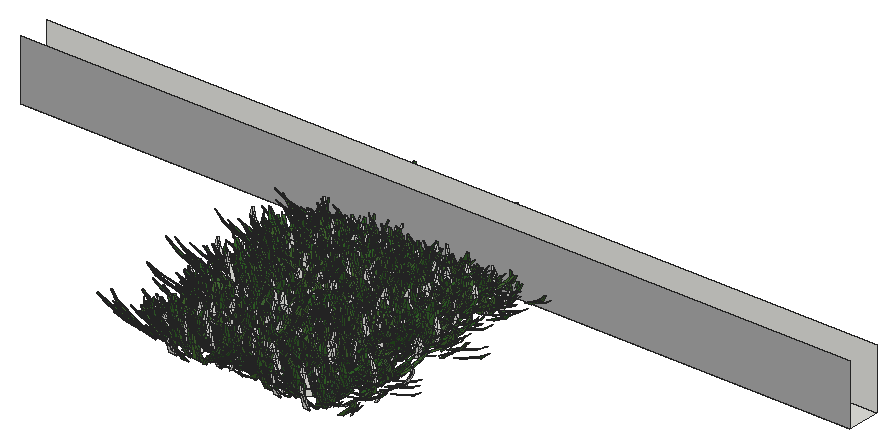
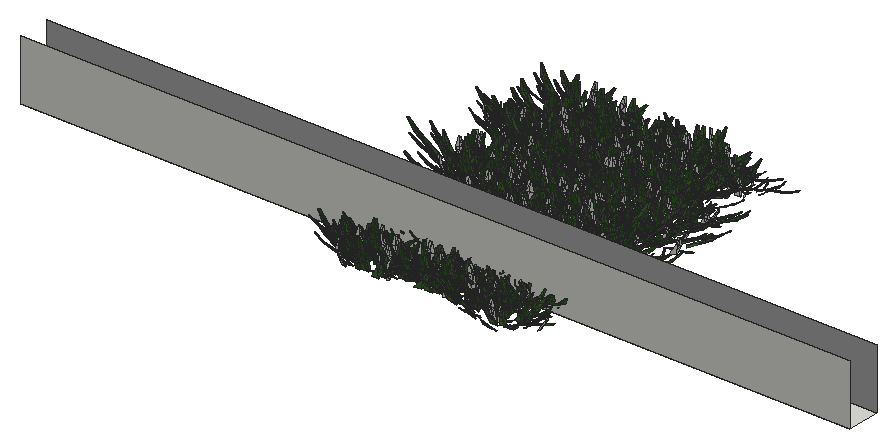
# SketchUp Ruby script. Lengths in inches.
U = 1.inch
M = Sketchup.active_model
def pt(a) = Geom::Point3d.new(a.map { |v| v * U })
def face(e, loops, mat)
  f = e.add_face(loops[0].map { |a| pt(a) })
  loops[1..].each { |l| e.add_face(l.map { |a| pt(a) }).erase! }
  f.material = f.back_material = mat if mat
  f
end
# faces: each face lists its corners as indices into pts; further lists are holes
def faces(e, pts, list, mat = nil) = list.each { |f| face(e, (f[0].is_a?(Array) ? f : [f]).map { |l| l.map { |i| pts[i] } }, mat) }
# xy, xz, yz: faces in a plane at the given z, y or x. An outline is a flat list of corners, or four numbers for a rectangle; further outlines are holes
def ring(l) = l.size == 4 ? [[l[0], l[1]], [l[2], l[1]], [l[2], l[3]], [l[0], l[3]]] : l.each_slice(2).to_a
def flat(e, list, mat, &to3) = list.each { |f| face(e, (f[0].is_a?(Array) ? f : [f]).map { |l| ring(l).map { |u, v| to3.(u, v) } }, mat) }
def xy(e, z, list, mat = nil) = flat(e, list, mat) { |x, y| [x, y, z] }
def xz(e, y, list, mat = nil) = flat(e, list, mat) { |x, z| [x, y, z] }
def yz(e, x, list, mat = nil) = flat(e, list, mat) { |y, z| [x, y, z] }
def lines(e, pts, list) = list.each { |a, b| e.add_line(pt(pts[a]), pt(pts[b])) }
# prism: a flat outline (further loops are holes) pulled along v
def prism(e, loops, v, mat = nil)
  f = face(e, loops, mat); d = Geom::Vector3d.new(v.map { |x| x * U })
  f.pushpull(f.normal.samedirection?(d) ? d.length : -d.length)
end
def box(e, o, s, mat = nil) = prism(e, [[o, [o[0] + s[0], o[1], o[2]], [o[0] + s[0], o[1] + s[1], o[2]], [o[0], o[1] + s[1], o[2]]]], [0, 0, s[2]], mat)
def at(x, y, z, deg = 0) = Geom::Transformation.translation(pt([x, y, z])) * Geom::Transformation.rotation(ORIGIN, Z_AXIS, deg.degrees)
def axes(o, x, y, z) = Geom::Transformation.new([*x, 0, *y, 0, *z, 0, *pt(o).to_a, 1])
def part(name) = M.definitions.add(name)
# library, detail: a bought-in or finely detailed component or shape, given as its bounding box
def library(name, o, s) = part(name).tap { |d| box(d.entities, o, s) }
def detail(e, o, s) = box(e.add_group.entities, o, s)
def put(e, d, t, mat = nil) = e.add_instance(d, t).tap { |i| i.material = mat if mat }
def group(e, t, mat = nil) = e.add_group.tap { |g| g.transformation = t; g.material = mat if mat }.entities
root = M.entities
M.materials.add("Material82").color = [68, 110, 58]
M.materials.add("Material83").color = [48, 90, 38]
M.materials.add("Material84").color = [68, 110, 48]
M.materials.add("Material85").color = [48, 90, 48]
M.materials.add("Material86").color = [58, 110, 58]
M.materials.add("Material87").color = [58, 90, 38]
M.materials.add("Material88").color = [68, 100, 58]
M.materials.add("Material89").color = [48, 100, 38]
M.materials.add("[Color M03]1").color = [170, 170, 170]
c1 = part("grass00")
p = [[-0.6875,0.15,0],[-0.56,0.08,5.52],[-0.04,0.03,2.76],[0.48,-0.02,0],[0.35,-0.02,5.52],[-0.1,-0.14,5.52],
  [-0.12,0.65,8.37],[-0.42,0.65,8.37]]
faces(c1.entities,p,[[0,1,2,3],[3,2,4],[1,5,2],[5,4,2],[1,6,5],[4,5,6],[7,6,1]])
c2 = part("Group16\#1")
put(c2.entities,c1,axes([1.44,-0.61,-0.01],[0.05352,0.12609,0],[-0.10704,0.04543,0.07239],[0.06664,-0.02828,0.11628]),"Material85")
put(c2.entities,c1,axes([0.76,-0.15,-0.01],[0.04676,0.24062,0],[-0.23162,0.04501,0.06642],[0.0652,-0.01267,0.23595]),"Material82")
put(c2.entities,c1,axes([0.79,0.01,-0.01],[-0.00606,0.34651,0],[-0.34381,-0.00602,0.0432],[0.04319,0.00076,0.34386]))
put(c2.entities,c1,axes([1,0.23,-0.01],[-0.07192,0.31144,0],[-0.28722,-0.06632,0.1236],[0.12043,0.02781,0.29478]),"Material84")
put(c2.entities,c1,axes([1.66,0.77,-0.01],[-0.13828,0.29651,0],[-0.21551,-0.1005,0.22471],[0.20365,0.09498,0.23779]),"Material89")
put(c2.entities,c1,axes([0.6875,0.52,-0.01],[-0.18126,0.24051,0],[-0.22746,-0.17142,0.09788],[0.07817,0.05891,0.28481]),"Material84")
put(c2.entities,c1,axes([0.68,0.78,-0.01],[-0.215,0.18688,0],[-0.12385,-0.14248,0.21334],[0.13995,0.16101,0.18878]),"Material82")
put(c2.entities,c1,axes([0.56,1,-0.01],[-0.13756,0.07624,0],[-0.06159,-0.11112,0.0927],[0.04494,0.08108,0.12705]),"Material84")
put(c2.entities,c1,axes([0.2,0.64,-0.01],[-0.23729,0.07254,0],[-0.05711,-0.18681,0.153],[0.04473,0.14632,0.19535]),"Material89")
put(c2.entities,c1,axes([0.0625,0.72,-0.01],[-0.28874,0.02525,0],[-0.02179,-0.24916,0.14647],[0.01276,0.14591,0.25012]),"Material82")
put(c2.entities,c1,axes([-0.08,0.62,-0.01],[-0.34089,-0.04187,0],[0.03255,-0.26504,0.216],[-0.02633,0.21439,0.26703]),"Material89")
put(c2.entities,c1,axes([-0.34,0.98,-0.01],[-0.14314,-0.0493,0],[0.04397,-0.12769,0.06843],[-0.02228,0.0647,0.13505]),"Material89")
put(c2.entities,c1,axes([-0.87,1.45,-0.01],[-0.23488,-0.14114,0],[0.13761,-0.22901,0.06087],[-0.03135,0.05217,0.26717]))
put(c2.entities,c1,axes([-0.72,0.77,-0.01],[-0.14208,-0.13251,0],[0.07209,-0.0773,0.16301],[-0.11118,0.11922,0.1057]),"Material89")
put(c2.entities,c1,axes([-0.62,0.43,-0.01],[-0.14845,-0.21203,0],[0.18654,-0.13061,0.12304],[-0.10079,0.07057,0.22772]),"Material82")
put(c2.entities,c1,axes([-0.68,0.29,-0.01],[-0.13639,-0.32136,0],[0.31723,-0.13464,0.05579],[-0.05136,0.0218,0.34462]),"Material83")
put(c2.entities,c1,axes([-0.64,0.125,-0.01],[-0.0458,-0.23569,0],[0.22124,-0.043,0.08276],[-0.08124,0.01579,0.22538]),"Material86")
put(c2.entities,c1,axes([-1.6,-0.03,-0.01],[0.00576,-0.32897,0],[0.27526,0.00482,0.18018],[-0.18015,-0.00315,0.2753]),"Material84")
put(c2.entities,c1,axes([-1.36,-0.31,-0.01],[0.05718,-0.24765,0],[0.18172,0.04196,0.17267],[-0.16825,-0.03885,0.1865]),"Material89")
put(c2.entities,c1,axes([-1.54,-0.72,-0.01],[0.06537,-0.14017,0],[0.13555,0.06321,0.03939],[-0.0357,-0.01665,0.14956]))
put(c2.entities,c1,axes([-1.19,-0.9,-0.01],[0.09597,-0.12735,0],[0.11214,0.08451,0.07557],[-0.06035,-0.04548,0.14042]),"Material88")
put(c2.entities,c1,axes([-0.47,-0.54,-0.01],[0.11588,-0.10072,0],[0.0618,0.0711,0.12124],[-0.07953,-0.0915,0.0942]))
put(c2.entities,c1,axes([-0.47,-0.84,-0.01],[0.11927,-0.0661,0],[0.06603,0.11913,0.00646],[-0.00313,-0.00565,0.13621]),"Material84")
put(c2.entities,c1,axes([-0.38,-1.24,-0.01],[0.28037,-0.08571,0],[0.0618,0.20215,0.20315],[-0.05939,-0.19428,0.21139]),"Material88")
put(c2.entities,c1,axes([-0.06,-0.66,-0.01],[0.22719,-0.01987,0],[0.01247,0.14255,0.17758],[-0.01547,-0.17691,0.1431]),"Material87")
put(c2.entities,c1,axes([0.11,-0.89,-0.01],[0.14882,0.01828,0],[-0.01058,0.08611,0.12229],[0.01491,-0.12138,0.08676]),"Material85")
put(c2.entities,c1,axes([0.25,-0.72,-0.01],[0.20481,0.07053,0],[-0.06206,0.18022,0.10291],[0.03351,-0.0973,0.1906]),"Material85")
put(c2.entities,c1,axes([0.85,-1.42,-0.01],[0.16481,0.09904,0],[-0.09472,0.15762,0.05616],[0.02893,-0.04814,0.18389]),"Material84")
put(c2.entities,c1,axes([1.01,-1.09,-0.01],[0.21858,0.20385,0],[-0.17495,0.1876,0.15339],[0.10462,-0.11218,0.25652]),"Material89")
put(c2.entities,c1,axes([1.01,-0.71,-0.01],[0.08733,0.12473,0],[-0.06445,0.04512,0.13037],[0.1068,-0.07477,0.07867]),"Material85")
c3 = part("Group15\#1")
put(c3.entities,c2,at(0,0,0))
c4 = part("3darcstudiotree_grass00\#1")
put(c4.entities,c3,at(0,0,0))
xy(root,-29.74,[[1674.65,1040.81,1830.75,1046.93]])
xz(root,1040.81,[[1674.65,-29.74,1830.75,-18.36]],"[Color M03]1")
xz(root,1046.93,[[1674.65,-29.74,1830.75,-18.36]])
put(root,c4,axes([1733.58,1045.64,-29.74],[3.16719,1.22877,0],[-2.37702,0.9529,-0.00671],[-0.02839,0.01138,1.53359]))
put(root,c4,axes([1733.55,1030.39,-29.74],[3.90875,0.99817,0],[-2.33451,1.4218,-0.02279],[-0.07245,0.04412,1.88252]))
put(root,c4,axes([1734.125,1020.67,-29.74],[4.17909,0.84834,0],[-2.02565,1.55199,-0.04224],[-0.09233,0.07074,1.58426]))
put(root,c4,axes([1734.54,1000.44,-29.74],[3.56991,0.07978,0],[-0.21949,1.52742,-0.02759],[-0.00848,0.05902,1.57942]))
put(root,c4,axes([1734.46,1053.28,-29.74],[1.29207,1.70529,0],[-3.1938,0.37636,-0.01522],[-0.08109,0.00956,1.38916]))
put(root,c4,axes([1736.35,1013.6,-29.74],[-4.32084,-0.18562,0],[0.42888,-1.55273,-0.0047],[0.00255,-0.00922,1.4854]))
put(root,c4,axes([1734.79,1027.98,-29.74],[0.16976,1.81896,0],[-4.60297,0.06681,-0.03073],[-0.13236,0.00192,1.48809]))
put(root,c4,axes([1736.42,1042.1,-29.74],[-3.93222,-0.02635,0],[0.07503,-1.74154,-0.03595],[0.00307,-0.07126,1.66434]))
put(root,c4,axes([1736.71,1030.11,-29.74],[-3.5417,-0.59044,0],[1.62012,-1.51145,-0.0473],[0.08471,-0.07903,1.43445]))
put(root,c4,axes([1734.9,1012.4,-29.74],[4.0668,0.76332,0],[-1.54133,1.27718,-0.01473],[-0.03515,0.02913,1.49308]))
put(root,c4,axes([1736.49,1016.9,-29.74],[-3.98791,0.79031,0],[-1.65069,-1.29546,-0.0516],[-0.1637,-0.12847,1.94674]))
put(root,c4,axes([1737.02,1020.82,-29.74],[-3.83726,0.13979,0],[-0.31883,-1.36117,-0.04806],[-0.027,-0.11528,1.58689]))
put(root,c4,axes([1736.78,1039.78,-29.74],[2.03121,-1.05332,0],[3.7313,1.11909,-0.04371],[0.13933,0.04179,1.40723]))
put(root,c4,axes([1737.75,1049.32,-29.74],[-3.73597,-0.76469,0],[1.79369,-1.36294,-0.02416],[0.05526,-0.04199,1.4491]))
put(root,c4,axes([1737.79,1046.82,-29.74],[-2.98813,-0.54786,0],[1.47052,-1.24742,-0.04575],[0.11826,-0.10032,1.60296]))
put(root,c4,axes([1736.7,1034.5,-29.74],[1.22817,1.22832,0],[-3.29828,0.51292,-0.04901],[-0.28268,0.04396,1.64754]))
put(root,c4,axes([1737.86,1009.17,-29.74],[-3.41944,0.15794,0],[-0.40533,-1.36487,-0.03745],[-0.0251,-0.08453,1.50509]))
put(root,c4,axes([1736.56,1003.46,-29.74],[0.51016,1.70246,0],[-4.00788,0.18679,-0.00527],[-0.02601,0.00121,1.50433]))
put(root,c4,axes([1737.16,1052.03,-29.74],[3.58477,-0.09461,0],[0.24683,1.45461,-0.02393],[0.00869,0.05119,1.50627]))
put(root,c4,axes([1737.03,1031.39,-29.74],[3.76255,0.21279,0],[-0.50611,1.39184,-0.02285],[-0.01632,0.04489,1.34478]))
put(root,c4,axes([1738.5,999.18,-29.74],[-4.15336,0.88478,0],[-2.07336,-1.51373,-0.03525],[-0.06704,-0.04895,1.3087]))
put(root,c4,axes([1738.67,1006.1,-29.74],[1.23783,-1.57966,0],[3.18362,0.388,-0.00928],[0.06663,0.00812,1.87692]))
put(root,c4,axes([1737.5,1018.83,-29.74],[4.18297,0.824,0],[-1.87304,1.47883,-0.04234],[-0.08644,0.06825,1.4356]))
put(root,c4,axes([1738.03,1038.62,-29.74],[3.73542,0.56333,0],[-1.36375,1.40645,-0.02441],[-0.06005,0.06193,1.97124]))
put(root,c4,axes([1738,1036.05,-29.74],[4.26727,0.66803,0],[-1.41698,1.40776,-0.04113],[-0.07249,0.07202,1.37498]))
put(root,c4,axes([1738.51,1044.36,-29.74],[1.59793,1.26945,0],[-3.48077,0.68144,-0.01001],[-0.04528,0.00886,1.4706]))
put(root,c4,axes([1740.36,1026.61,-29.74],[-4.24589,-0.20577,0],[0.52914,-1.69815,-0.04768],[0.02678,-0.08595,1.49744]))
put(root,c4,axes([1738.88,1011.83,-29.74],[0.88024,1.52698,0],[-4.39329,0.39388,-0.06457],[-0.26955,0.02417,1.44574]))
put(root,c4,axes([1739.9,1001.02,-29.74],[2.74133,-1.23391,0],[3.31507,1.14547,-0.04981],[0.18948,0.06547,1.67091]))
put(root,c4,axes([1739.01,1024.72,-29.74],[3.13752,1.05459,0],[-2.29496,1.06192,-0.00613],[-0.02513,0.01163,1.67562]))
put(root,c4,axes([1739.87,1006.93,-29.74],[1.5924,1.20755,0],[-3.44476,0.70651,-0.03549],[-0.1652,0.03388,1.52707]))
put(root,c4,axes([1739.65,1023.18,-29.74],[1.54833,1.52017,0],[-4.09421,0.64856,-0.00669],[-0.03642,0.00577,1.94122]))
put(root,c4,axes([1742.62,998.22,-29.74],[-1.94812,-1.05267,0],[3.13916,-0.90354,-0.00015],[0.00082,-0.00024,1.94435]))
put(root,c4,axes([1742.33,1022.625,-29.74],[-0.04856,-1.33378,0],[4.56796,-0.02587,-0.06189],[0.3016,-0.00171,1.66883]))
put(root,c4,axes([1742.66,1049.73,-29.74],[-2.95598,-0.91326,0],[2.43781,-1.22721,-0.04081],[0.12436,-0.0626,1.46417]))
put(root,c4,axes([1742.61,1040.13,-29.74],[-3.68784,-0.24252,0],[0.55953,-1.32329,-0.01602],[0.01459,-0.0345,1.41148]))
put(root,c4,axes([1743.21,1051.66,-29.74],[-0.4279,-1.35562,0],[4.45161,-0.21854,-0.05859],[0.31746,-0.01559,1.83593]))
put(root,c4,axes([1743.55,1029.53,-29.74],[-4.54384,0.18076,0],[-0.35947,-1.40543,-0.00469],[-0.00344,-0.01343,1.96044]))
put(root,c4,axes([1743.8,1031.91,-29.74],[-3.59063,0.36551,0],[-0.927,-1.41632,-0.03018],[-0.05381,-0.08221,1.98332]))
put(root,c4,axes([1744.3125,1046.29,-29.74],[-3.48173,-0.56284,0],[1.61416,-1.55298,-0.01809],[0.03189,-0.03068,1.4829]))
put(root,c4,axes([1743.78,1044.32,-29.74],[1.06749,-1.46896,0],[3.76494,0.42553,-0.03571],[0.22932,0.02592,1.9611]))
put(root,c4,axes([1743.9,1001.4,-29.74],[-3.26554,0.66263,0],[-1.53451,-1.17616,-0.01759],[-0.06154,-0.04717,1.92222]))
put(root,c4,axes([1743.68,1013.97,-29.74],[2.51439,-1.31879,0],[3.78,1.12088,-0.05965],[0.2657,0.07879,1.97549]))
put(root,c4,axes([1742.9,1036.05,-29.74],[4.03419,0.29669,0],[-0.75311,1.59264,-0.00417],[-0.00465,0.00984,1.87295]))
put(root,c4,axes([1744.47,1015.69,-29.74],[-0.70547,-1.57622,0],[3.40493,-0.23702,-0.01992],[0.12135,-0.00845,1.60321]))
put(root,c4,axes([1742.9,1009.8,-29.74],[4.47557,0.19067,0],[-0.50576,1.84642,-0.03307],[-0.01603,0.05854,1.59331]))
put(root,c4,axes([1743.32,1025.3,-29.74],[0.58274,1.76141,0],[-3.38049,0.17394,-0.03746],[-0.24477,0.01259,1.68385]))
put(root,c4,axes([1744.01,1007,-29.74],[-3.09447,0.74267,0],[-2.17746,-1.41107,-0.01391],[-0.03982,-0.0258,1.7292]))
put(root,c4,axes([1744.22,1011.56,-29.74],[2.464,-1.39681,0],[2.85004,0.78193,-0.02795],[0.16419,0.04505,1.86246]))
put(root,c4,axes([1743.9,1033.86,-29.74],[-1.9685,1.46825,0],[-4.07305,-0.84931,-0.01892],[-0.07094,-0.01479,1.46501]))
put(root,c4,axes([1745.63,1042.58,-29.74],[-2.90199,-1.04001,0],[2.97522,-1.29119,-0.02206],[0.0727,-0.03155,1.62457]))
put(root,c4,axes([1744.12,1019.07,-29.74],[-1.84293,1.54258,0],[-3.69335,-0.68627,-0.00165],[-0.00726,-0.00135,1.48801]))
put(root,c4,axes([1745.72,1002.77,-29.74],[-4.60496,-0.17881,0],[0.42059,-1.68464,-0.00134],[0.00055,-0.00219,1.33719]))
put(root,c4,axes([1743.84,1038.96,-29.74],[1.66114,1.62878,0],[-3.87747,0.61504,-0.0015],[-0.00686,0.00109,1.54039]))
put(root,c4,axes([1745.3,1005.53,-29.74],[2.67997,-1.42027,0],[3.59345,1.05458,-0.05496],[0.18586,0.05455,1.41537]))
put(root,c4,axes([1745.49,1020.51,-29.74],[0.63899,1.37464,0],[-4.27438,0.30902,-0.00804],[-0.04314,0.00312,1.77733]))
put(root,c4,axes([1745.73,1027.89,-29.74],[1.87438,1.56788,0],[-3.52749,0.65588,-0.03917],[-0.21764,0.04047,1.79585]))
put(root,c4,axes([1748.25,1003.08,-29.74],[-1.02752,-1.39563,0],[3.42384,-0.39205,-0.00444],[0.02976,-0.00341,1.86591]))
put(root,c4,axes([1747.68,1022.7,-29.74],[1.33366,-1.36849,0],[3.54112,0.53673,-0.03841],[0.22056,0.03343,1.74904]))
put(root,c4,axes([1748.15,1031.28,-29.74],[-1.96103,-1.06216,0],[3.43549,-0.98649,-0.06067],[0.27868,-0.08002,1.80988]))
put(root,c4,axes([1748.04,1007.51,-29.74],[-3.04968,0.59415,0],[-1.75652,-1.40223,-0.03032],[-0.06781,-0.05413,1.50108]))
put(root,c4,axes([1748.01,1038.84,-29.74],[3.38929,-0.88137,0],[2.3631,1.41334,-0.02666],[0.06787,0.04059,1.48784]))
put(root,c4,axes([1749.03,1051.15,-29.74],[0.25727,-1.4604,0],[3.98489,0.10918,-0.0172],[0.09613,0.00263,1.67763]))
put(root,c4,axes([1748.62,999.79,-29.74],[-2.6125,1.23987,0],[-2.75746,-0.90365,-0.04997],[-0.20997,-0.06881,1.46822]))
put(root,c4,axes([1749.71,1036.89,-29.74],[-3.77025,-0.95024,0],[2.35793,-1.45505,-0.05584],[0.17762,-0.10961,1.93872]))
put(root,c4,axes([1748.35,1006.09,-29.74],[-0.25979,1.36498,0],[-3.68566,-0.1091,-0.02554],[-0.15097,-0.00447,1.64241]))
put(root,c4,axes([1750.11,1011.36,-29.74],[-4.34871,0.30764,0],[-0.79873,-1.75601,-0.00093],[-0.00077,-0.00169,1.58752]))
put(root,c4,axes([1748.92,1001.57,-29.74],[3.80887,0.06416,0],[-0.18164,1.67717,-0.01987],[-0.00391,0.03608,1.47043]))
put(root,c4,axes([1748.95,1014.125,-29.74],[4.17174,-0.07865,0],[0.15922,1.3134,-0.03217],[0.01066,0.0879,1.73328]))
put(root,c4,axes([1749.14,1016.18,-29.74],[3.86863,-0.34225,0],[0.73265,1.28801,-0.00297],[0.00437,0.00768,1.68702]))
put(root,c4,axes([1750.83,1046.97,-29.74],[-2.85085,-0.66888,0],[2.41654,-1.60188,-0.00321],[0.00686,-0.00455,1.48019]))
put(root,c4,axes([1750.04,1039.84,-29.74],[-3.53825,1.08299,0],[-2.59336,-1.31776,-0.03049],[-0.10241,-0.05204,1.73706]))
put(root,c4,axes([1749.35,1025.99,-29.74],[3.26947,0.70015,0],[-1.66816,1.21153,-0.03457],[-0.12105,0.08791,1.92264]))
put(root,c4,axes([1750.3125,1045.13,-29.74],[2.00503,-1.14609,0],[3.00042,0.81639,-0.0362],[0.21042,0.05725,1.92943]))
put(root,c4,axes([1749.91,1010.31,-29.74],[-1.46805,1.46647,0],[-4.14161,-0.64484,-0.02576],[-0.10998,-0.01712,1.53201]))
put(root,c4,axes([1750,1018.24,-29.74],[4.25624,-0.01859,0],[0.03959,1.4097,-0.01976],[0.00112,0.03979,1.36845]))
put(root,c4,axes([1750.23,1029.43,-29.74],[2.49415,0.97261,0],[-2.31115,0.92177,-0.02576],[-0.13853,0.05525,1.88472]))
put(root,c4,axes([1750.33,1033.34,-29.74],[4.40385,0.48107,0],[-1.25638,1.78876,-0.02222],[-0.03253,0.04631,1.93436]))
put(root,c4,axes([1750.66,1049.27,-29.74],[2.4354,1.06288,0],[-2.86607,1.02137,-0.0306],[-0.14622,0.05211,1.86488]))
put(root,c4,axes([1751.45,1020.0625,-29.74],[-2.30622,1.23379,0],[-2.8482,-0.82802,-0.0238],[-0.11552,-0.03358,1.59896]))
put(root,c4,axes([1750.8,1043.29,-29.74],[1.42863,1.44478,0],[-4.37041,0.67213,-0.01645],[-0.07678,0.01181,1.76201]))
put(root,c4,axes([1751.07,1028.11,-29.74],[1.30118,1.34593,0],[-3.49846,0.52602,-0.01397],[-0.0708,0.01064,1.52193]))
put(root,c4,axes([1753.65,1001.875,-29.74],[-2.87014,-1.48867,0],[3.23188,-0.96911,-0.02],[0.09309,-0.02792,1.779]))
put(root,c4,axes([1753.42,1003.27,-29.74],[-0.3493,-1.81077,0],[4.63308,-0.139,-0.05882],[0.26935,-0.00808,1.5994]))
put(root,c4,axes([1753.8,1014.95,-29.74],[-3.58056,-0.39826,0],[0.95821,-1.33984,-0.015],[0.02011,-0.02812,1.30652]))
put(root,c4,axes([1752.99,1047.25,-29.74],[-0.87127,1.65753,0],[-3.69619,-0.30217,-0.02464],[-0.15319,-0.01252,1.79662]))
put(root,c4,axes([1753.65,1005.5625,-29.74],[-3.11874,1.35551,0],[-2.91461,-1.04296,-0.0082],[-0.03562,-0.01275,1.73071]))
put(root,c4,axes([1753.375,1045.39,-29.74],[-0.23965,1.40351,0],[-3.9598,-0.10516,-0.04305],[-0.25813,-0.00685,1.78778]))
put(root,c4,axes([1754.42,1028.82,-29.74],[-4.32286,0.64319,0],[-1.64772,-1.72238,-0.03096],[-0.05617,-0.05872,1.79846]))
put(root,c4,axes([1754.97,1012.73,-29.74],[-3.23633,-0.50825,0],[1.72306,-1.70642,-0.01803],[0.03469,-0.03435,1.81493]))
put(root,c4,axes([1753.89,1024.93,-29.74],[-1.77081,1.15286,0],[-3.98211,-0.9513,-0.05645],[-0.27396,-0.06545,1.97994]))
put(root,c4,axes([1755.23,1041.2,-29.74],[-1.58728,-1.19948,0],[3.58979,-0.73882,-0.00435],[0.01908,-0.00393,1.50222]))
put(root,c4,axes([1753.75,1023.25,-29.74],[2.97915,0.86965,0],[-2.38175,1.26898,-0.05487],[-0.15774,0.08404,1.44987]))
put(root,c4,axes([1753.84,1049.07,-29.74],[0.67536,1.71011,0],[-3.33591,0.2049,-0.00889],[-0.04851,0.00298,1.39664]))
put(root,c4,axes([1754.625,1051.69,-29.74],[2.58879,-1.26718,0],[2.80569,0.89147,-0.02709],[0.14156,0.04498,1.8123]))
put(root,c4,axes([1753.74,1036.52,-29.74],[3.8564,0.72862,0],[-1.8534,1.52567,-0.04599],[-0.08438,0.06946,1.36526]))
put(root,c4,axes([1755.8,1042.22,-29.74],[-3.19208,-0.59663,0],[1.68588,-1.40285,-0.03887],[0.08271,-0.06882,1.46596]))
put(root,c4,axes([1754.97,1021.08,-29.74],[3.36447,-1.00796,0],[2.1967,1.14039,-0.03309],[0.10605,0.05506,1.44206]))
put(root,c4,axes([1756.24,1031.47,-29.74],[-2.97002,-0.61033,0],[1.81963,-1.37718,-0.0201],[0.04091,-0.03096,1.30027]))
put(root,c4,axes([1756.42,1009.7,-29.74],[-3.57677,-1.09741,0],[2.84767,-1.44352,-0.06227],[0.15089,-0.07649,1.37168]))
put(root,c4,axes([1754.66,1038.09,-29.74],[1.39303,1.55232,0],[-3.39855,0.47433,-0.0171],[-0.11021,0.01538,1.84743]))
put(root,c4,axes([1755.29,999.38,-29.74],[-0.9025,1.72738,0],[-3.54084,-0.28772,-0.03296],[-0.16809,-0.01366,1.411]))
put(root,c4,axes([1755.45,1018.53,-29.74],[-1.59741,1.49736,0],[-3.22806,-0.5356,-0.02216],[-0.12937,-0.02146,1.66252]))
put(root,c4,axes([1756.47,1033.23,-29.74],[3.05945,-1.08948,0],[2.66485,1.16389,-0.04418],[0.16678,0.07284,1.67893]))
put(root,c4,axes([1756.23,1007.3,-29.74],[-0.7508,1.54691,0],[-4.43091,-0.33447,-0.01652],[-0.07223,-0.00545,1.50529]))
put(root,c4,axes([1756.42,1027.29,-29.74],[4.00478,-0.12141,0],[0.32544,1.66956,-0.03486],[0.01415,0.07259,1.68524]))
put(root,c4,axes([1756.82,1016.2,-29.74],[3.83024,1.03121,0],[-2.22146,1.2833,-0.02215],[-0.08012,0.04629,1.8946]))
put(root,c4,axes([1758.67,1031.82,-29.74],[0.46065,-1.85098,0],[4.3401,0.16799,-0.05803],[0.23131,0.00895,1.30918]))
put(root,c4,axes([1759.47,1036.35,-29.74],[-2.75759,-1.29294,0],[3.16062,-1.04842,-0.04595],[0.19898,-0.066,1.75181]))
put(root,c4,axes([1759,1038.98,-29.74],[2.18609,-1.17283,0],[3.5885,1.04029,-0.0227],[0.08817,0.02556,1.60931]))
put(root,c4,axes([1759.71,1012.24,-29.74],[-3.68156,-0.36216,0],[0.87025,-1.37591,-0.04204],[0.06138,-0.09705,1.62585]))
put(root,c4,axes([1759.37,998.85,-29.74],[-3.79448,1.12109,0],[-2.55555,-1.34526,-0.03017],[-0.0978,-0.05148,1.72726]))
put(root,c4,axes([1758.66,1034.34,-29.74],[1.1355,1.36945,0],[-3.88951,0.50159,-0.05705],[-0.27012,0.03483,1.52794]))
put(root,c4,axes([1760.35,1045.67,-29.74],[-3.52632,-0.01876,0],[0.05142,-1.50323,-0.03579],[0.00272,-0.07942,1.60809]))
put(root,c4,axes([1759.74,1023.05,-29.74],[-3.10715,1.0196,0],[-2.89034,-1.36991,-0.01948],[-0.06651,-0.03152,1.80807]))
put(root,c4,axes([1760,1052.16,-29.74],[-3.0378,0.91986,0],[-2.50548,-1.28689,-0.05552],[-0.17911,-0.092,1.63365]))
put(root,c4,axes([1758.85,1041.97,-29.74],[1.49785,1.29889,0],[-3.32043,0.59552,-0.00419],[-0.02419,0.00434,1.73548]))
put(root,c4,axes([1759.95,1020.54,-29.74],[3.31286,-0.55128,0],[1.80617,1.68812,-0.0407],[0.06877,0.06427,1.51351]))
put(root,c4,axes([1759.22,1001.96,-29.74],[3.22227,0.82324,0],[-2.17222,1.32236,-0.01048],[-0.0296,0.01802,1.55517]))
put(root,c4,axes([1761.36,1018.85,-29.74],[-4.269,-0.81813,0],[1.88917,-1.53314,-0.01545],[0.03796,-0.03081,1.8215]))
put(root,c4,axes([1759.22,1046.58,-29.74],[2.65644,1.45338,0],[-3.09672,0.88031,-0.01552],[-0.06337,0.01801,1.43977]))
put(root,c4,axes([1760.07,1014.21,-29.74],[0.15057,1.31453,0],[-3.70176,0.06595,-0.0329],[-0.23461,0.00418,1.98251]))
put(root,c4,axes([1760.04,1006.3,-29.74],[-0.68682,1.71759,0],[-4.33467,-0.26958,-0.03641],[-0.15889,-0.00988,1.45326]))
put(root,c4,axes([1760.13,1040.14,-29.74],[4.28771,-0.12133,0],[0.32919,1.80935,-0.01186],[0.00375,0.02059,1.52253]))
put(root,c4,axes([1760.92,1052.92,-29.74],[2.17543,-1.37172,0],[2.92508,0.72149,-0.0272],[0.16226,0.04002,1.81972]))
put(root,c4,axes([1760.46,1007.125,-29.74],[-1.33529,1.77622,0],[-3.16975,-0.37061,-0.00114],[-0.00828,-0.00097,1.86907]))
put(root,c4,axes([1759.99,1015.79,-29.74],[1.34239,1.63135,0],[-4.02681,0.51535,-0.01715],[-0.07258,0.00929,1.41194]))
put(root,c4,axes([1761.09,1025.18,-29.74],[-1.89402,1.2029,0],[-3.60721,-0.88336,-0.02009],[-0.09037,-0.02213,1.68525]))
put(root,c4,axes([1761.89,1027.93,-29.74],[-1.08101,1.66314,0],[-4.29936,-0.43462,-0.05431],[-0.26643,-0.02693,1.6847]))
put(root,c4,axes([1762.27,1049.39,-29.74],[-2.99935,1.42497,0],[-3.08029,-1.00838,-0.00469],[-0.01919,-0.00628,1.59556]))
put(root,c4,axes([1761.76,1029.88,-29.74],[2.63123,0.92373,0],[-2.85346,1.26414,-0.03405],[-0.11674,0.05172,1.65877]))
put(root,c4,axes([1762.02,1009.82,-29.74],[2.81192,0.87479,0],[-2.84329,1.42145,-0.06164],[-0.14998,0.07498,1.3518]))
put(root,c4,axes([1762.36,1003.16,-29.74],[0.48103,1.53156,0],[-4.51259,0.22043,-0.03401],[-0.13914,0.0068,1.40523]))
put(root,c4,axes([1764.47,1034.75,-29.74],[1.2731,-1.20941,0],[3.44603,0.56418,-0.03248],[0.17294,0.02831,1.61223]))
put(root,c4,axes([1764.85,1020.05,-29.74],[-3.65599,0.07986,0],[-0.21877,-1.55768,-0.04105],[-0.01403,-0.0999,1.83253]))
put(root,c4,axes([1764.02,1036.68,-29.74],[-0.67685,1.82709,0],[-3.63349,-0.20935,-0.03578],[-0.17247,-0.00994,1.34076]))
put(root,c4,axes([1764.87,998.26,-29.74],[-3.15287,0.69435,0],[-1.94177,-1.37131,-0.05669],[-0.17259,-0.12189,1.86391]))
put(root,c4,axes([1765.46,1009.83,-29.74],[-2.36391,-1.30666,0],[2.88424,-0.81154,-0.04134],[0.24623,-0.06928,1.943]))
put(root,c4,axes([1764.74,1004.16,-29.74],[-2.91503,0.96344,0],[-2.99535,-1.40954,-0.01682],[-0.05566,-0.02619,1.80026]))
put(root,c4,axes([1765.08,1042.3,-29.74],[-3.36658,1.12781,0],[-2.16506,-1.00516,-0.00331],[-0.01262,-0.00586,1.47415]))
put(root,c4,axes([1765.53,1008.5,-29.74],[2.5477,-1.31265,0],[2.99582,0.90433,-0.00025],[0.00104,0.00031,1.45509]))
put(root,c4,axes([1765.37,1022.9,-29.74],[2.84002,-1.42543,0],[3.17904,0.98511,-0.04001],[0.1906,0.05906,1.83572]))
